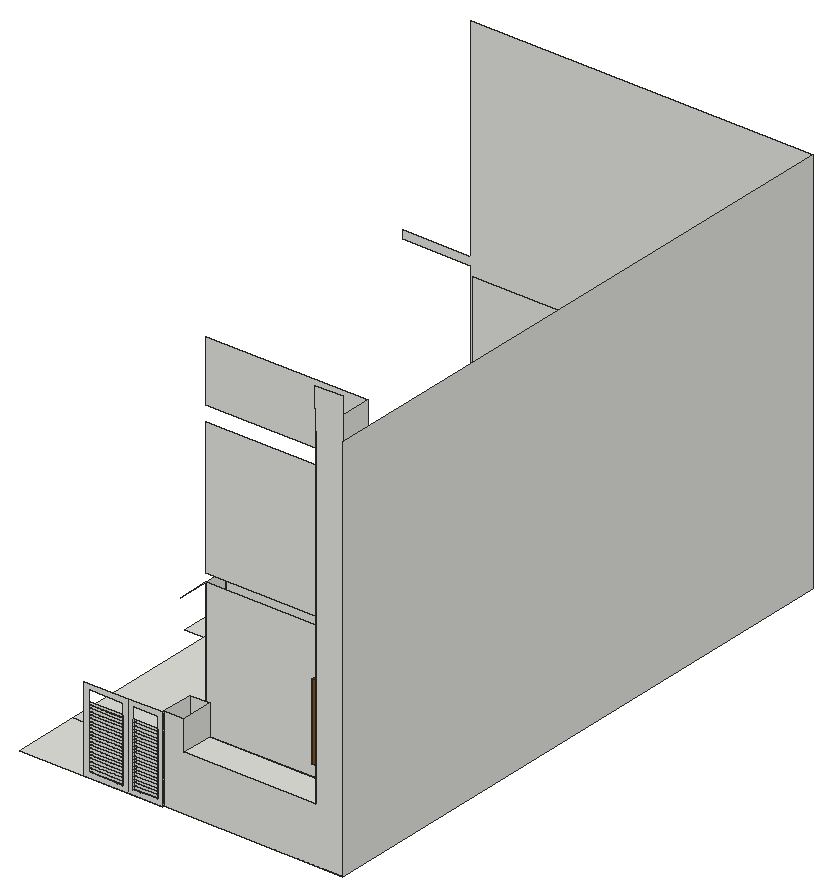
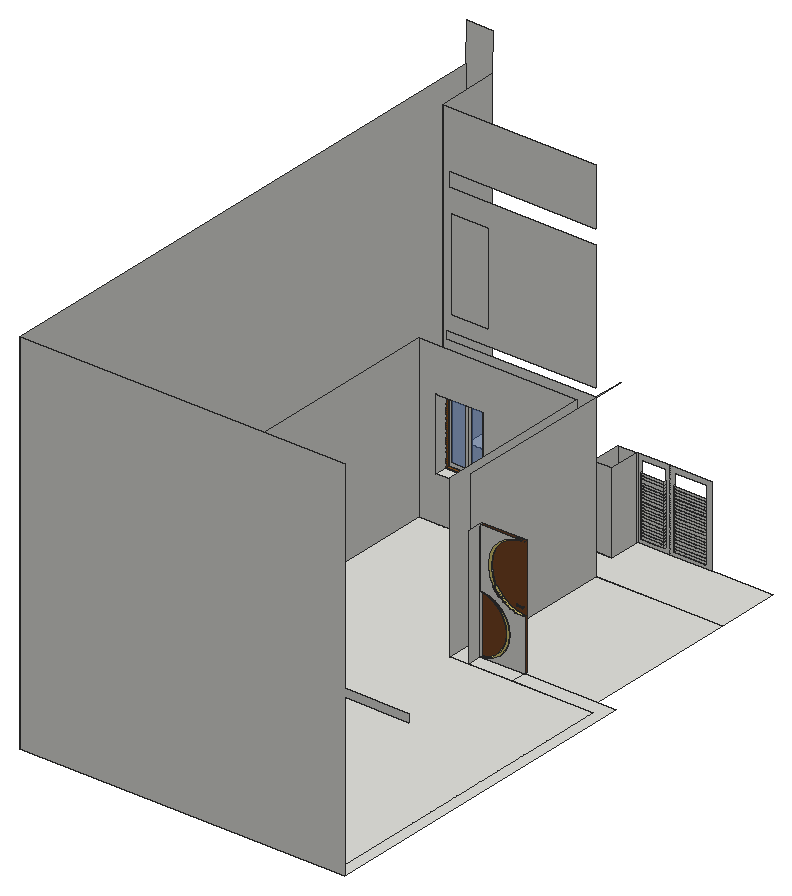
# SketchUp Ruby script. Lengths in inches.
U = 1.inch
M = Sketchup.active_model
def pt(a) = Geom::Point3d.new(a.map { |v| v * U })
def face(e, loops, mat)
  f = e.add_face(loops[0].map { |a| pt(a) })
  loops[1..].each { |l| e.add_face(l.map { |a| pt(a) }).erase! }
  f.material = f.back_material = mat if mat
  f
end
# faces: each face lists its corners as indices into pts; further lists are holes
def faces(e, pts, list, mat = nil) = list.each { |f| face(e, (f[0].is_a?(Array) ? f : [f]).map { |l| l.map { |i| pts[i] } }, mat) }
# xy, xz, yz: faces in a plane at the given z, y or x. An outline is a flat list of corners, or four numbers for a rectangle; further outlines are holes
def ring(l) = l.size == 4 ? [[l[0], l[1]], [l[2], l[1]], [l[2], l[3]], [l[0], l[3]]] : l.each_slice(2).to_a
def flat(e, list, mat, &to3) = list.each { |f| face(e, (f[0].is_a?(Array) ? f : [f]).map { |l| ring(l).map { |u, v| to3.(u, v) } }, mat) }
def xy(e, z, list, mat = nil) = flat(e, list, mat) { |x, y| [x, y, z] }
def xz(e, y, list, mat = nil) = flat(e, list, mat) { |x, z| [x, y, z] }
def yz(e, x, list, mat = nil) = flat(e, list, mat) { |y, z| [x, y, z] }
def lines(e, pts, list) = list.each { |a, b| e.add_line(pt(pts[a]), pt(pts[b])) }
# prism: a flat outline (further loops are holes) pulled along v
def prism(e, loops, v, mat = nil)
  f = face(e, loops, mat); d = Geom::Vector3d.new(v.map { |x| x * U })
  f.pushpull(f.normal.samedirection?(d) ? d.length : -d.length)
end
def box(e, o, s, mat = nil) = prism(e, [[o, [o[0] + s[0], o[1], o[2]], [o[0] + s[0], o[1] + s[1], o[2]], [o[0], o[1] + s[1], o[2]]]], [0, 0, s[2]], mat)
def at(x, y, z, deg = 0) = Geom::Transformation.translation(pt([x, y, z])) * Geom::Transformation.rotation(ORIGIN, Z_AXIS, deg.degrees)
def axes(o, x, y, z) = Geom::Transformation.new([*x, 0, *y, 0, *z, 0, *pt(o).to_a, 1])
def part(name) = M.definitions.add(name)
# library, detail: a bought-in or finely detailed component or shape, given as its bounding box
def library(name, o, s) = part(name).tap { |d| box(d.entities, o, s) }
def detail(e, o, s) = box(e.add_group.entities, o, s)
def put(e, d, t, mat = nil) = e.add_instance(d, t).tap { |i| i.material = mat if mat }
def group(e, t, mat = nil) = e.add_group.tap { |g| g.transformation = t; g.material = mat if mat }.entities
root = M.entities
M.materials.add("Teddy_SkinShadow ").color = [134, 77, 23]
M.materials.add("[Translucent Glass Blue]").color = [100, 149, 237]
M.materials["[Translucent Glass Blue]"].alpha = 0.5
M.materials.add("[Wood Bamboo]").color = [177, 105, 43]
M.materials.add("[Wood Board Cork]").color = [215, 201, 115]
M.materials.add("[Wood Veneer 01]").color = [120, 70, 37]
xy(root,0,[[1098.461,64.973,1199.684,64.973,1199.684,88.973,1307.818,88.973,1307.818,111.973,1098.461,111.973],[1199.684,65.973,1307.818,88.973],[1307.818,65.973,1327.309,111.973],[1192.934,111.973,1327.309,111.973,1327.309,482.785,1084.247,482.785,1084.247,229.266,1152.795,229.266,1152.795,240.054,1093.247,240.054,1093.247,473.785,1318.309,473.785,1318.309,120.973,1199.881,120.973,1199.881,240.054,1186.043,240.054,1186.043,229.266,1192.934,229.266],[1098.461,111.973,1192.934,111.973,1192.934,229.266,1186.043,229.266,1186.043,227.266,1152.795,227.266,1152.795,229.266,1098.461,229.266],
  [1199.881,120.973,1318.309,120.973,1318.309,473.785,1093.247,473.785,1093.247,240.054,1199.881,240.054],[1152.795,227.266,1186.043,229.266],[1152.795,229.266,1186.043,240.054]])
xy(root,3.559,[[1147.452,64.973,1171.711,65.973],[1178.83,64.973,1186.173,65.973],[1186.173,64.973,1196.125,65.973]])
xy(root,33.064,[[1270.891,111.973,1305.742,120.973]])
xy(root,33.064,[[1270.891,108.973,1305.742,111.973]],"Teddy_SkinShadow ")
xy(root,35.648,[[1273.474,108.973,1288.316,111.973],[1288.316,108.973,1303.158,111.973]],"Teddy_SkinShadow ")
xy(root,39.125,[[1213.899,65.973,1307.818,88.973]])
xy(root,42.3125,[[1155.396,226.016,1160.008,227.266]],"[Wood Bamboo]")
xy(root,43.5,[[1155.396,226.016,1160.008,227.266]],"[Wood Bamboo]")
xz(root,64.973,[[[1143.893,0,1175.271,60],[1147.452,3.559,1171.711,56.441]],[[1175.271,0,1199.684,60],[1178.83,3.559,1196.125,56.441]]])
xz(root,65.973,[[1199.684,0,1327.309,0,1327.309,276.1875,1326.739,305.307,1307.248,304.925,1307.818,275.806,1307.818,39.125,1213.899,39.125,1213.899,60.1875,1199.684,60.1875],[1147.452,3.559,1171.711,3.622],[1178.83,3.559,1196.125,5.673],[1147.452,3.622,1171.711,5.734],[1178.83,5.673,1196.125,5.675],
  [1178.83,5.675,1196.125,7.788],[1147.452,5.734,1171.711,5.753],[1147.452,5.753,1171.711,7.846],[1178.83,7.788,1196.125,7.79],[1178.83,7.79,1196.125,9.903],
  [1147.452,7.846,1171.711,7.865],[1147.452,7.865,1171.711,9.958],[1178.83,9.903,1196.125,9.905],[1178.83,9.905,1196.125,12.019],[1147.452,9.958,1171.711,9.977],
  [1147.452,9.977,1171.711,12.07],[1178.83,12.019,1196.125,12.021],[1178.83,12.021,1196.125,14.134],[1147.452,12.07,1171.711,12.089],[1147.452,12.089,1171.711,14.182],
  [1178.83,14.134,1196.125,14.136],[1178.83,14.136,1196.125,16.249],[1147.452,14.182,1171.711,14.201],[1147.452,14.201,1171.711,16.294],[1178.83,16.249,1196.125,16.251],
  [1178.83,16.251,1196.125,18.365],[1147.452,16.294,1171.711,16.313],[1147.452,16.313,1171.711,18.406],[1178.83,18.365,1196.125,18.367],[1178.83,18.367,1196.125,20.48],
  [1147.452,18.406,1171.711,18.425],[1147.452,18.425,1171.711,20.518],[1178.83,20.48,1196.125,20.482],[1178.83,20.482,1196.125,22.595],[1147.452,20.518,1171.711,20.537],
  [1147.452,20.537,1171.711,22.63],[1178.83,22.595,1196.125,22.597],[1178.83,22.597,1196.125,24.711],[1147.452,22.63,1171.711,22.649],[1147.452,22.649,1171.711,24.742],
  [1178.83,24.711,1196.125,24.713],[1178.83,24.713,1196.125,26.826],[1147.452,24.742,1171.711,24.761],[1147.452,24.761,1171.711,26.854],[1178.83,26.826,1196.125,26.828],
  [1178.83,26.828,1196.125,28.941],[1147.452,26.854,1171.711,26.873],[1147.452,26.873,1171.711,28.966],[1178.83,28.941,1196.125,28.943],[1178.83,28.943,1196.125,31.057],
  [1147.452,28.966,1171.711,28.985],[1147.452,28.985,1171.711,31.078],[1178.83,31.057,1196.125,31.059],[1178.83,31.059,1196.125,33.172],[1147.452,31.078,1171.711,31.097],
  [1147.452,31.097,1171.711,33.19],[1178.83,33.172,1196.125,33.174],[1178.83,33.174,1196.125,35.287],[1147.452,33.19,1171.711,33.209],[1147.452,33.209,1171.711,35.302],
  [1178.83,35.287,1196.125,35.289],[1178.83,35.289,1196.125,37.403],[1147.452,35.302,1171.711,35.321],[1147.452,35.321,1171.711,37.414],[1178.83,37.403,1196.125,37.405],
  [1178.83,37.405,1196.125,39.518],[1147.452,37.414,1171.711,37.433],[1147.452,37.433,1171.711,39.526],[1178.83,39.518,1196.125,39.52],[1178.83,39.52,1196.125,41.633],
  [1147.452,39.526,1171.711,39.545],[1147.452,39.545,1171.711,41.638],[1178.83,41.633,1196.125,41.635],[1178.83,41.635,1196.125,43.749],[1147.452,41.638,1171.711,41.657],
  [1147.452,41.657,1171.711,43.75],[1178.83,43.749,1196.125,43.751],[1147.452,43.75,1171.711,43.769],[1178.83,43.751,1196.125,45.864],[1147.452,43.769,1171.711,45.862],
  [1147.452,45.862,1171.711,45.881],[1178.83,45.864,1196.125,45.866],[1178.83,45.866,1196.125,47.979],[1147.452,45.881,1171.711,47.974]])
xz(root,88.973,[[1199.684,0,1213.899,60.1875],[1213.899,0,1307.818,39.125]])
xz(root,108.973,[[[1270.891,33.064,1305.742,86.936],[1273.474,35.648,1303.158,84.352]]],"Teddy_SkinShadow ")
xz(root,111.973,[[[1192.934,0,1307.818,0,1307.818,275.806,1192.934,275.806,1192.934,232.677,1303.381,232.677,1303.381,222,1192.934,222,1192.934,126,1305.309,126,1305.309,119.9375,1192.934,119.9375],[1273.529,137.022,1301.638,205.381],[1270.891,33.064,1305.742,86.936]],[[1273.474,35.648,1288.316,84.352],[1275.66,37.833,1286.131,82.167]],[[1288.316,35.648,1303.158,84.352],[1290.501,37.833,1300.973,82.167]]])
xz(root,111.973,[[1275.66,37.833,1286.131,82.167],[1290.501,37.833,1300.973,82.167]],"[Translucent Glass Blue]")
xz(root,120.973,[[[1199.881,0,1318.309,120],[1270.891,33.064,1305.742,86.936]]])
xz(root,226.016,[[1154.758,42.031,1154.985,42.061,1155.196,42.148,1155.377,42.287,1155.396,42.3125,1160.008,42.3125,1160.008,43.5,1155.396,43.5,1155.377,43.525,1155.196,43.664,1154.985,43.751,1154.758,43.781,1154.532,43.751,1154.321,43.664,1154.139,43.525,1154,43.344,1153.913,43.133,1153.883,42.906,1153.913,42.68,1154,42.469,1154.139,42.287,1154.321,42.148,1154.532,42.061]],"[Wood Bamboo]")
xz(root,227.266,[[1152.795,0,1186.043,0,1180.29,0.757,1174.929,2.978,1170.325,6.511,1166.792,11.115,1164.571,16.476,1163.814,22.23,1164.571,27.983,1166.792,33.345,1170.325,37.949,1174.929,41.481,1180.29,43.702,1186.043,44.46,1186.043,88.919,1152.795,88.919,1159.715,88.48,1166.259,86.185,1171.937,82.203,1176.326,76.834,1179.097,70.477,1180.045,63.607,1179.097,56.737,1176.326,50.38,1171.937,45.011,1166.259,41.029,1159.715,38.733,1152.795,38.294],[1186.043,0,1186.043,44.46,1180.79,43.179,1175.997,40.677,1171.944,37.098,1168.867,32.652,1166.946,27.597,1166.293,22.23,1166.946,16.862,1168.867,11.808,1171.944,7.362,1175.997,3.783,1180.79,1.28],[[1152.795,38.294,1159.346,39.157,1165.451,41.686,1170.693,45.708,1174.716,50.951,1177.245,57.056,1178.107,63.607,1177.245,70.158,1174.716,76.263,1170.693,81.506,1165.451,85.528,1159.346,88.057,1152.795,88.919],[1154.758,42.031,1154.532,42.061,1154.321,42.148,1154.139,42.287,1154,42.469,1153.913,42.68,1153.883,42.906,1153.913,43.133,1154,43.344,1154.139,43.525,1154.321,43.664,1154.532,43.751,1154.758,43.781,1154.985,43.751,1155.196,43.664,1155.377,43.525,1155.396,43.5,1160.008,43.5,1160.008,42.3125,1155.396,42.3125,1155.377,42.287,1155.196,42.148,1154.985,42.061]]],"[Wood Veneer 01]")
xz(root,229.266,[[1152.795,0,1186.043,0,1180.29,0.757,1174.929,2.978,1170.325,6.511,1166.792,11.115,1164.571,16.476,1163.814,22.23,1164.571,27.983,1166.792,33.345,1170.325,37.949,1174.929,41.481,1180.29,43.702,1186.043,44.46,1186.043,88.919,1152.795,88.919,1159.715,88.48,1166.259,86.185,1171.937,82.203,1176.326,76.834,1179.097,70.477,1180.045,63.607,1179.097,56.737,1176.326,50.38,1171.937,45.011,1166.259,41.029,1159.715,38.733,1152.795,38.294]])
xz(root,229.266,[[1186.043,0,1180.79,1.28,1175.997,3.783,1171.944,7.362,1168.867,11.808,1166.946,16.862,1166.293,22.23,1166.946,27.597,1168.867,32.652,1171.944,37.098,1175.997,40.677,1180.79,43.179,1186.043,44.46,1180.29,43.702,1174.929,41.481,1170.325,37.949,1166.792,33.345,1164.571,27.983,1163.814,22.23,1164.571,16.476,1166.792,11.115,1170.325,6.511,1174.929,2.978,1180.29,0.757],[1152.795,38.294,1159.715,38.733,1166.259,41.029,1171.937,45.011,1176.326,50.38,1179.097,56.737,1180.045,63.607,1179.097,70.477,1176.326,76.834,1171.937,82.203,1166.259,86.185,1159.715,88.48,1152.795,88.919,1159.346,88.057,1165.451,85.528,1170.693,81.506,1174.716,76.263,1177.245,70.158,1178.107,63.607,1177.245,57.056,1174.716,50.951,1170.693,45.708,1165.451,41.686,1159.346,39.157]],"[Wood Board Cork]")
xz(root,473.785,[[1093.247,0,1318.309,120]])
xz(root,482.785,[[1084.247,0,1084.247,120,1036.059,120,1036.059,126,1084.247,126,1084.247,276.1875,1327.309,276.1875,1327.309,0]])
yz(root,1160.008,[[226.016,42.3125,227.266,43.5]],"[Wood Bamboo]")
yz(root,1171.711,[[64.973,3.559,65.973,3.622],[64.973,3.622,65.973,5.734],[64.973,5.734,65.973,5.753],[64.973,5.753,65.973,7.846],[64.973,7.846,65.973,7.865],
  [64.973,7.865,65.973,9.958],[64.973,9.958,65.973,9.977],[64.973,9.977,65.973,12.07],[64.973,12.07,65.973,12.089],[64.973,12.089,65.973,14.182],
  [64.973,14.182,65.973,14.201],[64.973,14.201,65.973,16.294],[64.973,16.294,65.973,16.313],[64.973,16.313,65.973,18.406],[64.973,18.406,65.973,18.425],
  [64.973,18.425,65.973,20.518],[64.973,20.518,65.973,20.537],[64.973,20.537,65.973,22.63],[64.973,22.63,65.973,22.649],[64.973,22.649,65.973,24.742],
  [64.973,24.742,65.973,24.761],[64.973,24.761,65.973,26.854],[64.973,26.854,65.973,26.873],[64.973,26.873,65.973,28.966],[64.973,28.966,65.973,28.985],
  [64.973,28.985,65.973,31.078],[64.973,31.078,65.973,31.097],[64.973,31.097,65.973,33.19],[64.973,33.19,65.973,33.209],[64.973,33.209,65.973,35.302],
  [64.973,35.302,65.973,35.321],[64.973,35.321,65.973,37.414],[64.973,37.414,65.973,37.433],[64.973,37.433,65.973,39.526],[64.973,39.526,65.973,39.545],
  [64.973,39.545,65.973,41.638],[64.973,41.638,65.973,41.657],[64.973,41.657,65.973,43.75],[64.973,43.75,65.973,43.769],[64.973,43.769,65.973,45.862],
  [64.973,45.862,65.973,45.881],[64.973,45.881,65.973,47.974]])
yz(root,1178.83,[[64.973,3.559,65.973,5.673],[64.973,5.673,65.973,5.675],[64.973,5.675,65.973,7.788],[64.973,7.788,65.973,7.79],[64.973,7.79,65.973,9.903],
  [64.973,9.903,65.973,9.905],[64.973,9.905,65.973,12.019],[64.973,12.019,65.973,12.021],[64.973,12.021,65.973,14.134],[64.973,14.134,65.973,14.136],
  [64.973,14.136,65.973,16.249],[64.973,16.249,65.973,16.251],[64.973,16.251,65.973,18.365],[64.973,18.365,65.973,18.367],[64.973,18.367,65.973,20.48],
  [64.973,20.48,65.973,20.482],[64.973,20.482,65.973,22.595],[64.973,22.595,65.973,22.597],[64.973,22.597,65.973,24.711],[64.973,24.711,65.973,24.713],
  [64.973,24.713,65.973,26.826],[64.973,26.826,65.973,26.828],[64.973,26.828,65.973,28.941],[64.973,28.941,65.973,28.943],[64.973,28.943,65.973,31.057],
  [64.973,31.057,65.973,31.059],[64.973,31.059,65.973,33.172],[64.973,33.172,65.973,33.174],[64.973,33.174,65.973,35.287],[64.973,35.287,65.973,35.289],
  [64.973,35.289,65.973,37.403],[64.973,37.403,65.973,37.405],[64.973,37.405,65.973,39.518],[64.973,39.518,65.973,39.52],[64.973,39.52,65.973,41.633],
  [64.973,41.633,65.973,41.635],[64.973,41.635,65.973,43.749],[64.973,43.749,65.973,43.751],[64.973,43.751,65.973,45.864],[64.973,45.864,65.973,45.866],
  [64.973,45.866,65.973,47.979]])
yz(root,1186.043,[[227.266,0,229.266,44.46],[229.266,0,240.054,88.919],[227.266,44.46,229.266,88.919]])
yz(root,1192.934,[[111.973,0,111.973,119.9375,89.348,119.9375,89.348,120,229.266,120,229.266,0]])
yz(root,1196.125,[[64.973,3.559,65.973,5.673],[64.973,5.673,65.973,5.675],[64.973,5.675,65.973,7.788],[64.973,7.788,65.973,7.79],[64.973,7.79,65.973,9.903],
  [64.973,9.903,65.973,9.905],[64.973,9.905,65.973,12.019],[64.973,12.019,65.973,12.021],[64.973,12.021,65.973,14.134],[64.973,14.134,65.973,14.136],
  [64.973,14.136,65.973,16.249],[64.973,16.249,65.973,16.251],[64.973,16.251,65.973,18.365],[64.973,18.365,65.973,18.367],[64.973,18.367,65.973,20.48],
  [64.973,20.48,65.973,20.482],[64.973,20.482,65.973,22.595],[64.973,22.595,65.973,22.597],[64.973,22.597,65.973,24.711],[64.973,24.711,65.973,24.713],
  [64.973,24.713,65.973,26.826],[64.973,26.826,65.973,26.828],[64.973,26.828,65.973,28.941],[64.973,28.941,65.973,28.943],[64.973,28.943,65.973,31.057],
  [64.973,31.057,65.973,31.059],[64.973,31.059,65.973,33.172],[64.973,33.172,65.973,33.174],[64.973,33.174,65.973,35.287],[64.973,35.287,65.973,35.289],
  [64.973,35.289,65.973,37.403],[64.973,37.403,65.973,37.405],[64.973,37.405,65.973,39.518],[64.973,39.518,65.973,39.52],[64.973,39.52,65.973,41.633],
  [64.973,41.633,65.973,41.635],[64.973,41.635,65.973,43.749],[64.973,43.749,65.973,43.751],[64.973,43.751,65.973,45.864],[64.973,45.864,65.973,45.866],
  [64.973,45.866,65.973,47.979]])
yz(root,1199.684,[[64.973,0,65.973,60],[65.973,0,88.973,60.1875]])
yz(root,1199.881,[[120.973,0,240.054,120]])
yz(root,1213.899,[[65.973,39.125,88.973,60.1875]])
yz(root,1270.891,[[111.973,33.064,120.973,86.936]])
yz(root,1270.891,[[108.973,33.064,111.973,86.936]],"Teddy_SkinShadow ")
yz(root,1273.474,[[108.973,35.648,111.973,84.352]],"Teddy_SkinShadow ")
yz(root,1303.158,[[108.973,35.648,111.973,84.352]],"Teddy_SkinShadow ")
yz(root,1305.742,[[111.973,33.064,120.973,86.936]])
yz(root,1305.742,[[108.973,33.064,111.973,86.936]],"Teddy_SkinShadow ")
yz(root,1307.818,[[88.973,0,88.973,39.125,65.973,39.125,65.973,275.806,111.973,275.806,111.973,0]])
yz(root,1318.309,[[120.973,0,473.785,120]])
yz(root,1327.309,[[65.973,0,482.785,276.1875]])
p = [[1186.043,229.266,0],[1180.29,229.266,0.757],[1180.29,227.266,0.757],[1186.043,227.266,0],[1180.79,229.266,1.28],[1180.79,227.266,1.28],
  [1174.929,229.266,2.978],[1174.929,227.266,2.978],[1175.997,229.266,3.783],[1175.997,227.266,3.783],[1170.325,229.266,6.511],[1170.325,227.266,6.511],
  [1171.944,229.266,7.362],[1171.944,227.266,7.362],[1166.792,229.266,11.115],[1166.792,227.266,11.115],[1168.867,229.266,11.808],[1168.867,227.266,11.808],
  [1164.571,229.266,16.476],[1164.571,227.266,16.476],[1166.946,229.266,16.862],[1166.946,227.266,16.862],[1163.814,229.266,22.23],[1163.814,227.266,22.23],
  [1166.293,229.266,22.23],[1166.293,227.266,22.23],[1164.571,229.266,27.983],[1164.571,227.266,27.983],[1166.946,229.266,27.597],[1166.946,227.266,27.597],
  [1168.867,229.266,32.652],[1168.867,227.266,32.652],[1166.792,229.266,33.345],[1166.792,227.266,33.345],[1171.944,229.266,37.098],[1171.944,227.266,37.098],
  [1170.325,229.266,37.949],[1170.325,227.266,37.949],[1175.997,229.266,40.677],[1175.997,227.266,40.677],[1174.929,229.266,41.481],[1174.929,227.266,41.481],
  [1152.795,229.266,38.294],[1159.346,229.266,39.157],[1159.346,227.266,39.157],[1152.795,227.266,38.294],[1159.715,229.266,38.733],[1159.715,227.266,38.733],
  [1166.259,229.266,41.029],[1166.259,227.266,41.029],[1165.451,229.266,41.686],[1165.451,227.266,41.686],[1180.79,229.266,43.179],[1180.79,227.266,43.179],
  [1171.937,229.266,45.011],[1171.937,227.266,45.011],[1180.29,229.266,43.702],[1180.29,227.266,43.702],[1170.693,229.266,45.708],[1170.693,227.266,45.708],
  [1154.532,227.266,42.061],[1154.758,227.266,42.031],[1154.758,226.016,42.031],[1154.532,226.016,42.061],[1154.985,227.266,42.061],[1154.985,226.016,42.061],
  [1154.139,227.266,42.287],[1154.321,227.266,42.148],[1154.321,226.016,42.148],[1154.139,226.016,42.287],[1155.196,227.266,42.148],[1155.196,226.016,42.148],
  [1155.377,227.266,42.287],[1155.377,226.016,42.287],[1155.396,227.266,42.3125],[1155.396,226.016,42.3125],[1186.043,229.266,44.46],[1186.043,227.266,44.46],
  [1154.321,227.266,43.664],[1154.139,227.266,43.525],[1154.139,226.016,43.525],[1154.321,226.016,43.664],[1155.377,227.266,43.525],[1155.196,227.266,43.664],
  [1155.196,226.016,43.664],[1155.377,226.016,43.525],[1155.396,227.266,43.5],[1155.396,226.016,43.5],[1154.532,227.266,43.751],[1154.532,226.016,43.751],
  [1154.985,227.266,43.751],[1154.985,226.016,43.751],[1154.758,227.266,43.781],[1154.758,226.016,43.781],[1176.326,229.266,50.38],[1176.326,227.266,50.38],
  [1174.716,229.266,50.951],[1174.716,227.266,50.951]]
faces(root,p,[[0,1,2,3],[4,0,3,5],[1,6,7,2],[8,4,5,9],[6,10,11,7],[12,8,9,13],[10,14,15,11],[16,12,13,17],
  [14,18,19,15],[20,16,17,21],[18,22,23,19],[24,20,21,25],[22,26,27,23],[28,24,25,29],[30,28,29,31],[26,32,33,27],
  [34,30,31,35],[32,36,37,33],[38,34,35,39],[36,40,41,37],[42,43,44,45],[46,42,45,47],[48,46,47,49],[43,50,51,44],
  [52,38,39,53],[54,48,49,55],[40,56,57,41],[50,58,59,51],[76,52,53,77],[56,76,77,57],[94,54,55,95],[58,96,97,59]],"[Wood Board Cork]")
faces(root,p,[[60,61,62,63],[61,64,65,62],[66,67,68,69],[67,60,63,68],[64,70,71,65],[70,72,73,71],[72,74,75,73],[78,79,80,81],
  [82,83,84,85],[86,82,85,87],[88,78,81,89],[83,90,91,84],[92,88,89,93],[90,92,93,91]],"[Wood Bamboo]")
